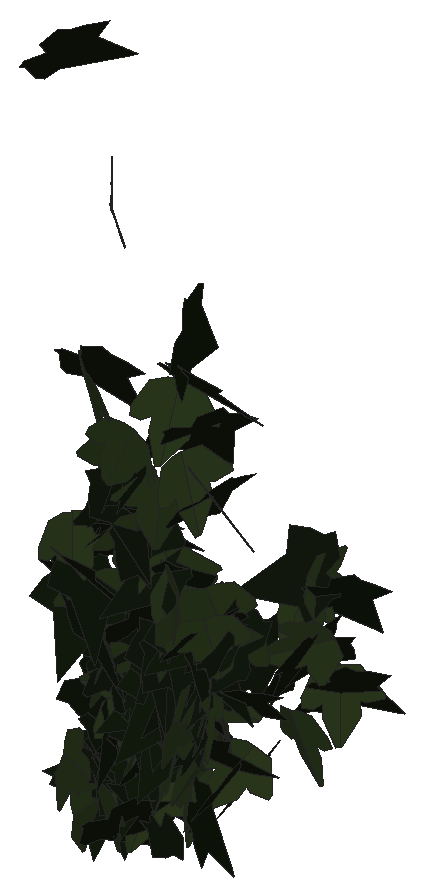
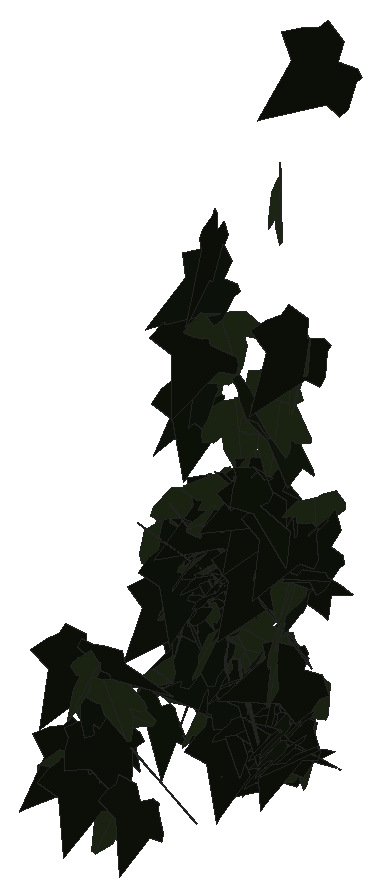
# SketchUp Ruby script. Lengths in inches.
U = 1.inch
M = Sketchup.active_model
def pt(a) = Geom::Point3d.new(a.map { |v| v * U })
def face(e, loops, mat)
  f = e.add_face(loops[0].map { |a| pt(a) })
  loops[1..].each { |l| e.add_face(l.map { |a| pt(a) }).erase! }
  f.material = f.back_material = mat if mat
  f
end
# faces: each face lists its corners as indices into pts; further lists are holes
def faces(e, pts, list, mat = nil) = list.each { |f| face(e, (f[0].is_a?(Array) ? f : [f]).map { |l| l.map { |i| pts[i] } }, mat) }
# xy, xz, yz: faces in a plane at the given z, y or x. An outline is a flat list of corners, or four numbers for a rectangle; further outlines are holes
def ring(l) = l.size == 4 ? [[l[0], l[1]], [l[2], l[1]], [l[2], l[3]], [l[0], l[3]]] : l.each_slice(2).to_a
def flat(e, list, mat, &to3) = list.each { |f| face(e, (f[0].is_a?(Array) ? f : [f]).map { |l| ring(l).map { |u, v| to3.(u, v) } }, mat) }
def xy(e, z, list, mat = nil) = flat(e, list, mat) { |x, y| [x, y, z] }
def xz(e, y, list, mat = nil) = flat(e, list, mat) { |x, z| [x, y, z] }
def yz(e, x, list, mat = nil) = flat(e, list, mat) { |y, z| [x, y, z] }
def lines(e, pts, list) = list.each { |a, b| e.add_line(pt(pts[a]), pt(pts[b])) }
# prism: a flat outline (further loops are holes) pulled along v
def prism(e, loops, v, mat = nil)
  f = face(e, loops, mat); d = Geom::Vector3d.new(v.map { |x| x * U })
  f.pushpull(f.normal.samedirection?(d) ? d.length : -d.length)
end
def box(e, o, s, mat = nil) = prism(e, [[o, [o[0] + s[0], o[1], o[2]], [o[0] + s[0], o[1] + s[1], o[2]], [o[0], o[1] + s[1], o[2]]]], [0, 0, s[2]], mat)
def at(x, y, z, deg = 0) = Geom::Transformation.translation(pt([x, y, z])) * Geom::Transformation.rotation(ORIGIN, Z_AXIS, deg.degrees)
def axes(o, x, y, z) = Geom::Transformation.new([*x, 0, *y, 0, *z, 0, *pt(o).to_a, 1])
def part(name) = M.definitions.add(name)
# library, detail: a bought-in or finely detailed component or shape, given as its bounding box
def library(name, o, s) = part(name).tap { |d| box(d.entities, o, s) }
def detail(e, o, s) = box(e.add_group.entities, o, s)
def put(e, d, t, mat = nil) = e.add_instance(d, t).tap { |i| i.material = mat if mat }
def group(e, t, mat = nil) = e.add_group.tap { |g| g.transformation = t; g.material = mat if mat }.entities
root = M.entities
M.materials.add("efeu1").color = [18, 25, 13]
M.materials.add("efeu2").color = [43, 57, 29]
c1 = part("ivyleaf_9")
p = [[1.54,2.16,1.25],[1.36,2.04,1.19],[-0.21,0.99,0.68],[-0.71,1.11,0.82],[-0.85,0.86,0.67],[-0.8,0.17,0.21],
  [-0.9,-0.01,0.1],[-0.67,-0.16,-0.02],[-0.08,-0.08,-0.05],[-0.03,-0.6,-0.4],[0.65,-0.88,-0.66],[0.83,-0.6,-0.49],
  [1.29,-0.42,-0.43],[1.8125,-0.07,-0.26],[1.21,0.44,0.15]]
faces(c1.entities,p,[[0,1,2,3,4,5,6,7,8,9,10,11,12,13,14]],"efeu1")
c2 = part("ivyleaf_10")
p = [[0,0.5,-0.03],[-0.0625,2.02,-0.43],[-0.19,2.01,-0.46],[-0.54,1.05,-0.29],[-0.52,0.625,-0.18],[-0.83,0.76,-0.28],
  [-1.16,0.64,-0.33],[-1.15,0.33,-0.24],[-0.77,-0.39,0.02],[-0.3,-0.51,0.16],[0.04,-0.48,0.23],[-0.02,2.01,-0.4375],
  [-0.06,2.01,-0.43],[0.04,-0.49,0.23],[0.67,-0.49,0.14],[1.38,0.36,-0.2],[1.375,0.51,-0.24],[0.81,0.65,-0.19],
  [0.62,0.59,-0.15],[0.6,1.09,-0.28],[0.5,1.23,-0.31]]
faces(c2.entities,p,[[0,1,2,3,4,5,6,7,8,9,10],[11,12,0,13,14,15,16,17,18,19,20]],"efeu2")
put(root,c1,axes([550.1,133.2,216.78],[-0.59429,0.6691,-0.0104],[0.00821,-0.00662,-0.89492],[-0.66913,-0.59434,-0.00174]))
put(root,c2,axes([551.52,132.83,210.04],[0.00997,-0.53866,-0.7302],[0.04576,0.72962,-0.5376],[0.90623,-0.03091,0.03518]))
put(root,c2,axes([547.84,132.95,207.55],[0.22412,-0.63918,-0.5683],[0.16925,0.60901,-0.61823],[0.83838,0.04792,0.27672]))
put(root,c2,axes([549.48,133.23,217.26],[0.81363,-0.00082,-0.37135],[-0.35071,0.29233,-0.76905],[0.12208,0.84524,0.26562]))
put(root,c1,axes([547.52,132.63,228.19],[0.59662,0.59328,0.51411],[0.32166,0.40429,-0.83984],[-0.71611,0.67588,0.05108]))
put(root,c1,axes([547.84,133.76,212.79],[0.12009,-0.87259,0.06119],[0.0064,-0.06088,-0.88081],[0.87471,0.12024,-0.00195]))
put(root,c2,axes([547.61,133.42,213.96],[0.41476,0.7663,-0.07857],[-0.02634,-0.07508,-0.87126],[-0.76987,0.41541,-0.01252]))
put(root,c2,axes([550.85,133.52,218.91],[0.769,0.44717,-0.1306],[-0.09655,-0.0936,-0.88898],[-0.45573,0.77437,-0.03204]))
put(root,c2,axes([550.43,133.52,216.05],[-0.64695,-0.6021,0.11233],[-0.02269,-0.13972,-0.87957],[0.61207,-0.64159,0.08613]))
put(root,c2,axes([548.34,133.16,218.72],[-0.70764,0.48513,0.2721],[-0.21416,0.16873,-0.8578],[-0.51335,-0.73914,-0.01723]))
put(root,c1,axes([551.33,133.11,219.97],[0.89887,-0.03814,0.0874],[0.09261,0.15182,-0.88625],[0.02271,0.89026,0.15488]))
put(root,c2,axes([551.38,133.3125,217.08],[0.29493,0.83891,0.11528],[0.01473,0.11697,-0.8889],[-0.84666,0.29426,0.02469]))
put(root,c1,axes([548.78,133.75,215.45],[0.34099,-0.82183,-0.03042],[0.05134,0.05414,-0.88715],[0.82079,0.33803,0.06813]))
put(root,c2,axes([549.48,133.65,214.68],[-0.18582,-0.86964,0.05641],[0.02343,-0.06264,-0.88855],[0.87115,-0.18381,0.03593]))
put(root,c1,axes([549.19,132.99,206.28],[0.42964,0.74315,0.1304],[0.06722,0.11176,-0.8584],[-0.7515,0.43486,-0.00223]))
put(root,c1,axes([549.125,132.9375,215.49],[0.02505,0.69432,0.56069],[-0.32716,0.52901,-0.64047],[-0.83031,-0.18749,0.26927]))
put(root,c2,axes([551.03,133.2,213.36],[0.44166,-0.37291,-0.65544],[-0.32638,0.59023,-0.55574],[0.67981,0.52565,0.15902]))
put(root,c1,axes([551.04,133.65,210.64],[-0.77046,0.36327,-0.14568],[0.13792,-0.04903,-0.85169],[-0.36629,-0.78258,-0.01426]))
put(root,c1,axes([550.57,133.79,213.86],[-0.86638,0.11673,0.05794],[-0.06172,-0.02448,-0.87361],[-0.11478,-0.86797,0.03243]))
put(root,c1,axes([551.59,132.99,221.29],[0.13884,-0.01392,-1.00697],[-0.8046,0.60978,-0.11937],[0.60564,0.81329,0.07226]))
put(root,c2,axes([548.91,133.57,216.54],[-0.87203,-0.15999,0.0083],[-0.00367,-0.02598,-0.88623],[0.16016,-0.87168,0.02489]))
put(root,c2,axes([551.89,133.59,212.45],[-0.66501,-0.522,-0.17987],[0.19529,0.041,-0.84098],[0.51643,-0.68768,0.0864]))
put(root,c1,axes([550.5625,134.05,210.05],[-0.78552,-0.34598,0.03958],[-0.03803,-0.01185,-0.85833],[0.34615,-0.78643,-0.00448]))
put(root,c1,axes([547.15,133.42,212.79],[0.84719,-0.09249,0.25483],[0.25779,0.01608,-0.85118],[0.08389,0.88454,0.04212]))
put(root,c1,axes([551.7,133.4,207.35],[0.52038,-0.38329,-0.62649],[-0.52649,0.34064,-0.64572],[0.51206,0.73976,-0.02726]))
put(root,c2,axes([548.47,133.57,206.54],[-0.68974,0.46227,-0.04073],[0.03183,-0.02565,-0.83032],[-0.46297,-0.69047,0.00358]))
put(root,c1,axes([547.54,133.91,211.3],[0.53574,-0.67289,0.13481],[0.07547,-0.11221,-0.86005],[0.6821,0.54093,-0.01072]))
put(root,c1,axes([548.09,133.32,219.18],[0.85039,0.33248,-0.06095],[-0.05712,-0.02127,-0.91307],[-0.33316,0.8523,0.00099]))
put(root,c1,axes([550.14,134.1875,211.12],[0.00544,-0.85844,0.11648],[0.02162,-0.11631,-0.85821],[0.86603,0.0083,0.0207]))
put(root,c1,axes([547.59,134.15,211.99],[-0.66488,-0.50789,-0.24826],[0.24612,0.08498,-0.83298],[0.50893,-0.70461,0.07849]))
put(root,c1,axes([549.45,133.7,214.47],[0.41913,-0.66792,-0.41325],[-0.20446,0.35948,-0.78838],[0.75835,0.46607,0.01585]))
put(root,c2,axes([549.05,133.33,223.87],[-0.31573,0.22129,0.83082],[-0.68853,0.465,-0.3855],[-0.51493,-0.75744,0.00606]))
put(root,c1,axes([550.84,134.35,211.76],[-0.13977,-0.85048,0.09091],[-0.00068,-0.09201,-0.86177],[0.85533,-0.13905,0.01417]))
put(root,c1,axes([551.02,134.48,210.72],[-0.35071,-0.75138,0.22692],[0.00049,-0.24876,-0.82291],[0.7849,-0.33558,0.10191]))
put(root,c2,axes([550.54,133.77,209.9],[0.49557,-0.67511,-0.30872],[-0.0493,0.34044,-0.82362],[0.74071,0.47434,0.15173]))
put(root,c2,axes([550.22,134.03,208.02],[0.61784,-0.591,-0.00668],[-0.00244,0.00712,-0.85499],[0.59104,0.61784,0.00346]))
put(root,c1,axes([552.07,133.98,212.36],[-0.78092,0.37303,0.01141],[-0.01345,-0.00168,-0.86541],[-0.37297,-0.781,0.00731]))
put(root,c1,axes([551.44,133.69,216.7],[0.83799,-0.20634,-0.25437],[-0.23718,0.09964,-0.86216],[0.2259,0.87006,0.03841]))
put(root,c1,axes([551.75,134.35,212.3],[-0.83264,-0.13282,0.17577],[-0.14592,-0.18234,-0.82902],[0.16506,-0.83122,0.15377]))
put(root,c2,axes([551.22,134.09,210.69],[0.71131,-0.45927,0.00572],[0.00622,-0.00091,-0.84669],[0.45927,0.71133,0.00261]))
put(root,c1,axes([548.14,134.52,208.2],[0.07675,-0.13064,-0.83273],[0.69945,-0.45676,0.13612],[-0.4704,-0.7005,0.06654]))
put(root,c1,axes([551.98,133.79,207.7],[-0.35239,0.76153,-0.1147],[0.06608,-0.09578,-0.83888],[-0.76728,-0.358,-0.01957]))
put(root,c1,axes([550.61,133.91,211.5],[0.0824,-0.6793,-0.52361],[-0.08807,0.51654,-0.68398],[0.85315,0.11894,-0.02004]))
put(root,c2,axes([547.89,133.32,205.97],[0.14147,-0.15741,-0.87203],[0.04387,0.88323,-0.15232],[0.88503,-0.01862,0.14694]))
put(root,c1,axes([551.67,133.65,212.3],[-0.01132,0.85999,-0.10711],[-0.06975,-0.10767,-0.85717],[-0.86383,-0.00258,0.07062]))
put(root,c1,axes([550.36,134.3,209.95],[-0.82343,-0.04598,0.22969],[-0.22557,-0.07081,-0.82281],[0.06319,-0.85193,0.05599]))
put(root,c1,axes([550.3,134.49,210.67],[-0.16176,-0.83823,0.10063],[-0.00217,-0.10205,-0.85352],[0.84424,-0.16087,0.01709]))
put(root,c1,axes([551.51,133.49,218.26],[0.47918,0.76139,0.02592],[0.00869,0.02515,-0.89961],[-0.76178,0.47922,0.00604]))
put(root,c1,axes([550.25,134.52,208.89],[-0.45574,-0.69815,0.11065],[-0.04309,-0.10397,-0.83348],[0.70555,-0.45731,0.02057]))
put(root,c2,axes([550.73,133.28,212.67],[0.05369,0.07302,-0.95829],[0.25136,0.92531,0.08459],[0.92762,-0.25496,0.03254]))
put(root,c2,axes([547.96,134,212.23],[-0.66066,-0.5489,-0.16054],[0.20403,0.00292,-0.84964],[0.53426,-0.67987,0.12596]))
put(root,c1,axes([550.17,134.47,210.16],[-0.43852,-0.7312,-0.11466],[0.07568,0.08828,-0.8524],[0.73626,-0.44458,0.01932]))
put(root,c2,axes([551.07,134.55,208.38],[0.08698,-0.66053,0.52545],[0.03316,-0.52515,-0.66565],[0.84339,0.08877,-0.02802]))
put(root,c2,axes([550.43,133.86,213.62],[0.65303,0.48624,0.35895],[0.15552,0.37548,-0.79155],[-0.58403,0.64367,0.19059]))
put(root,c1,axes([550.65,134.47,211.08],[-0.00442,-0.85306,-0.12076],[-0.0096,0.1208,-0.85301],[0.86151,-0.00303,-0.01012]))
put(root,c1,axes([551.67,133.6,216.15],[0.1781,0.86314,0.16315],[-0.05692,0.17746,-0.8767],[-0.87657,0.16385,0.09008]))
put(root,c1,axes([551.33,134.08,209.12],[-0.62846,0.56719,-0.00148],[0.00789,0.00654,-0.8465],[-0.56713,-0.62843,-0.01014]))
put(root,c2,axes([551.28,134.44,210],[-0.57612,0.44534,-0.42847],[0.10117,-0.50991,-0.66602],[-0.60965,-0.50546,0.29438]))
put(root,c2,axes([551.55,134.15,213],[-0.68929,-0.48487,-0.23796],[0.24681,0.06042,-0.83802],[0.48043,-0.7267,0.0891]))
put(root,c2,axes([550.76,133.97,211.49],[0.2504,0.79694,0.21061],[-0.10721,0.24973,-0.81751],[-0.8173,0.21141,0.17176]))
put(root,c1,axes([549.57,134.32,208.61],[0.66771,-0.50134,0.05059],[0.03826,-0.0333,-0.83497],[0.50244,0.6688,-0.00365]))
put(root,c2,axes([549.35,134.33,209.78],[0.30391,0.03428,-0.94877],[-0.94783,0.06804,-0.30115],[0.0544,0.99393,0.05334]))
put(root,c1,axes([549.1,134.66,207.64],[-0.63862,-0.48621,-0.27967],[0.30194,0.05916,-0.79233],[0.47271,-0.69466,0.12827]))
put(root,c1,axes([550.18,133.89,213.17],[0.84526,0.24851,0.29573],[0.28438,0.08117,-0.88103],[-0.26142,0.89181,-0.00222]))
put(root,c1,axes([548.66,134.55,209.31],[0.43421,-0.73922,0.02209],[0.04519,0.00095,-0.85641],[0.73817,0.43477,0.03943]))
put(root,c1,axes([548.57,133.96,210.19],[-0.31401,0.55915,0.59705],[-0.40628,0.44846,-0.63367],[-0.70997,-0.50394,0.09855]))
put(root,c2,axes([549.31,134.45,206.55],[0.58398,0.57092,-0.23145],[-0.2071,-0.11842,-0.81464],[-0.5802,0.61691,0.05783]))
put(root,c1,axes([548.55,133.91,214.34],[0.77845,0.22839,0.34224],[0.30181,0.18081,-0.80715],[-0.27964,0.83092,0.08157]))
put(root,c1,axes([548.9,134.06,214.53],[-0.1385,0.86615,-0.01475],[-0.15656,-0.03972,-0.86228],[-0.85201,-0.1335,0.16085]))
put(root,c1,axes([551.28,134.25,211.4],[0.50272,-0.52836,-0.45355],[-0.27329,0.3648,-0.7279],[0.64046,0.5704,0.04541]))
put(root,c1,axes([550.45,134.59,210.34],[-0.29929,-0.69263,-0.40311],[0.15995,0.37002,-0.75453],[0.78527,-0.33935,0.00005]))
put(root,c2,axes([548.79,134.29,208.75],[0.69716,0.4648,0.13844],[0.03667,0.19121,-0.82664],[-0.48359,0.68457,0.1369]))
put(root,c2,axes([551.18,134.37,209.46],[0.38891,-0.73348,-0.18883],[0.03357,0.22875,-0.81942],[0.75666,0.36686,0.13341]))
put(root,c2,axes([549.16,134.65,208.47],[0.38392,-0.73868,0.14378],[0.08519,-0.11771,-0.83223],[0.7477,0.3927,0.02099]))
put(root,c2,axes([552.05,134.52,211.92],[-0.75253,-0.30302,0.26361],[-0.21738,-0.16347,-0.80848],[0.33772,-0.78043,0.067]))
put(root,c2,axes([548.03,134.15,211.09],[-0.50428,0.65155,0.2966],[-0.17417,0.24023,-0.82386],[-0.69437,-0.53344,-0.00875]))
put(root,c1,axes([552.41,134.4,211.6],[-0.54561,0.49114,0.42681],[-0.46474,0.09571,-0.70423],[-0.45541,-0.68608,0.2073]))
put(root,c1,axes([547.41,134.91,206.29],[-0.21861,-0.807,-0.0371],[0.09937,0.01128,-0.83091],[0.80171,-0.22145,0.09287]))
put(root,c1,axes([549.14,134.875,208.41],[-0.05797,-0.84044,-0.02442],[0.01511,0.02343,-0.84233],[0.84066,-0.05837,0.01346]))
put(root,c1,axes([549.49,134.99,205.48],[0.21272,-0.79979,-0.11355],[0.02051,-0.11204,0.82755],[-0.80755,-0.21352,-0.0089]))
put(root,c2,axes([549.7,134.6,209.33],[-0.60687,-0.60003,0.03088],[0.09161,-0.13579,-0.83812],[0.5938,-0.59229,0.16086]))
put(root,c1,axes([548.45,134.625,206.625],[-0.61675,0.23153,0.49701],[-0.51172,0.02557,-0.64691],[-0.1969,-0.79167,0.12446]))
put(root,c1,axes([550.75,134.15,208.33],[0.75454,0.12845,0.38636],[0.35921,0.17302,-0.75904],[-0.19168,0.82986,0.09845]))
put(root,c1,axes([548.64,134.1,214.11],[0.69192,0.53596,0.01849],[0.00311,0.02618,-0.87502],[-0.53627,0.69167,0.01879]))
put(root,c1,axes([547.65,134.75,207.13],[0.15631,-0.78722,-0.26729],[-0.02489,0.26742,-0.80216],[0.83099,0.15608,0.02625]))
put(root,c1,axes([549.04,134.01,211.61],[0.39175,0.7292,0.29822],[0.11819,0.27489,-0.82741],[-0.77891,0.40846,0.02444]))
put(root,c2,axes([550.96,134.35,209.91],[0.50445,-0.38406,-0.67799],[-0.43002,0.53634,-0.62376],[0.64982,0.65306,0.11355]))
put(root,c2,axes([548.67,134.83,207.54],[0.3836,-0.73576,0.02906],[0.01255,-0.02624,-0.82975],[0.73623,0.3838,-0.001]))
put(root,c2,axes([550.24,134.83,208.09],[-0.38849,-0.14463,0.9129],[-0.8636,-0.29611,-0.41442],[0.3294,-0.9469,-0.00984]))
put(root,c2,axes([549.85,134.68,209.05],[0.83084,-0.10721,0.01454],[0.03612,0.16876,-0.81989],[0.10198,0.81365,0.17197]))
put(root,c1,axes([547.87,134.1,213.53],[0.36212,0.75936,0.24923],[0.09475,0.2309,-0.84118],[-0.79358,0.37407,0.0133]))
put(root,c1,axes([548.85,134.34,208.26],[0.10223,0.83622,-0.0593],[-0.00584,-0.05903,-0.84245],[-0.8383,0.10239,-0.00137]))
put(root,c2,axes([550.83,134.48,209.92],[-0.3319,-0.22153,-0.74813],[0.71009,0.25115,-0.38939],[0.32333,-0.77896,0.08722]))
put(root,c2,axes([551.37,134.6,209.95],[-0.52339,0.66157,0.02309],[-0.02687,0.00818,-0.84342],[-0.66142,-0.52383,0.01599]))
put(root,c1,axes([547.65,135.05,206.39],[0.0813,-0.82454,-0.07831],[-0.00181,0.07851,-0.82852],[0.82825,0.08111,0.00587]))
put(root,c1,axes([547.8125,134.37,207.11],[0.63302,0.53677,-0.22177],[-0.21654,-0.08626,-0.82686],[-0.53891,0.66518,0.07174]))
put(root,c1,axes([547.52,134.8,207.56],[0.57448,-0.61904,-0.04635],[0.07485,0.13177,-0.83212],[0.61625,0.56109,0.14428]))
put(root,c2,axes([547.94,134.52,209.76],[0.11758,-0.72401,-0.44865],[0.0687,0.45949,-0.7235],[0.84898,0.06309,0.12069]))
put(root,c1,axes([548.65,135.01,207.31],[-0.11508,-0.77726,-0.26],[0.06637,0.25285,-0.78526],[0.8169,-0.13004,0.02717]))
put(root,c1,axes([547.62,134.85,206.91],[0.58377,-0.60833,-0.00442],[0.09577,0.09795,-0.83193],[0.60076,0.57552,0.13692]))
put(root,c1,axes([549.54,134.46,207.65],[0.04038,0.83589,-0.07013],[0.01237,-0.0708,-0.83671],[-0.83873,0.0392,-0.01572]))
put(root,c2,axes([550.09,134.83,209.18],[-0.14294,0.81426,-0.16283],[0.00075,-0.1651,-0.82626],[-0.83038,-0.14032,0.02729]))
put(root,c2,axes([550.33,134.97,206.98],[-0.03897,0.78274,-0.29062],[-0.02699,-0.29196,-0.78274],[-0.83451,-0.02711,0.03889]))
put(root,c1,axes([547.35,134.41,209.1],[0.06559,0.16208,-0.84665],[0.31919,0.78418,0.17485],[0.80075,-0.32586,-0.00034]))
put(root,c2,axes([551.66,135.28,207.86],[0.51511,0.41241,-0.51416],[-0.38991,-0.33546,-0.6597],[-0.53142,0.64588,-0.01434]))
put(root,c1,axes([550.1,135.5,208.72],[0.83295,-0.54876,0.10469],[-0.06676,0.08883,0.99677],[-0.55465,-0.83479,0.03724]))
put(root,c1,axes([551.65,134.52,209.98],[0.69642,0.46459,0.12241],[-0.00024,0.21591,-0.81806],[-0.48045,0.67333,0.17785]))
put(root,c1,axes([551.32,134.66,211.28],[0.20436,0.81878,0.07955],[-0.01467,0.08558,-0.84318],[-0.82251,0.20191,0.0348]))
put(root,c1,axes([548.32,135.04,205.88],[0.31067,-0.0639,0.77088],[0.75987,-0.13014,-0.31702],[0.14465,0.82087,0.00975]))
put(root,c2,axes([549.8125,134.67,209.22],[-0.06259,0.06884,-0.8475],[-0.3457,0.77433,0.08843],[0.77685,0.35012,-0.02893]))
put(root,c1,axes([549.17,134.99,208.08],[0.63838,-0.11524,0.5274],[0.53984,0.13923,-0.62301],[-0.00195,0.81626,0.18073]))
put(root,c1,axes([549.16,135.1,206.49],[0.3826,0.73048,-0.09898],[-0.04725,-0.08698,-0.82461],[-0.73564,0.3855,0.00149]))
put(root,c1,axes([551.48,135.63,206.9375],[-0.12346,0.75644,0.33418],[-0.0777,0.32578,-0.76612],[-0.82331,-0.14418,0.02219]))
put(root,c2,axes([550.83,139.35,209.16],[0.22862,0.28388,-0.78081],[-0.78882,-0.18003,-0.29642],[-0.26079,0.79342,0.21211]))
put(root,c1,axes([550.74,139.22,209.26],[-0.3439,0.6801,-0.39933],[0.143,-0.37465,-0.76122],[-0.7756,-0.37063,0.03672]))
put(root,c1,axes([548.85,139.79,208.02],[-0.77257,0.30855,0.01572],[-0.02148,-0.01141,-0.8317],[-0.3082,-0.77265,0.01856]))
put(root,c1,axes([550.5,139.95,210.84],[-0.73477,0.04713,0.43865],[-0.43858,0.01411,-0.73618],[-0.0477,-0.85563,0.01202]))
put(root,c2,axes([549.78,139.9,206.23],[-0.78807,0.25492,-0.22503],[0.20503,-0.0969,-0.8278],[-0.27127,-0.81382,0.02807]))
put(root,c2,axes([549.76,140.07,210.11],[0.83875,0.05762,-0.139],[-0.13928,-0.00058,-0.84068],[-0.05694,0.85019,0.00885]))
put(root,c1,axes([550.1875,140,208.55],[0.03742,0.71147,-0.43043],[-0.21964,-0.4071,-0.69201],[-0.80201,0.14468,0.16944]))
put(root,c1,axes([551.01,139.69,210.66],[0.65797,0.53032,-0.0035],[-0.00034,-0.00516,-0.84508],[-0.53033,0.65796,-0.0038]))
put(root,c2,axes([550.72,140.35,207.58],[0.64423,0.53007,0.03919],[0.03268,0.02196,-0.83426],[-0.53051,0.64504,-0.0038]))
put(root,c2,axes([550.47,139.84,210.6],[-0.10438,0.60674,0.59736],[-0.15058,0.57919,-0.61459],[-0.83803,-0.17965,0.03603]))
put(root,c1,axes([550.8125,140.05,207.7],[0.67644,0.44561,0.20761],[0.16067,0.13335,-0.80972],[-0.4646,0.6949,0.02225]))
put(root,c1,axes([548.64,140.18,206.83],[0.09772,0.77027,0.27647],[0.02625,0.27534,-0.7764],[-0.81797,0.10086,0.00811]))
put(root,c1,axes([550.37,140.37,207.17],[0.31898,0.76835,0.04389],[-0.01598,0.05411,-0.83118],[-0.76944,0.31741,0.03545]))
